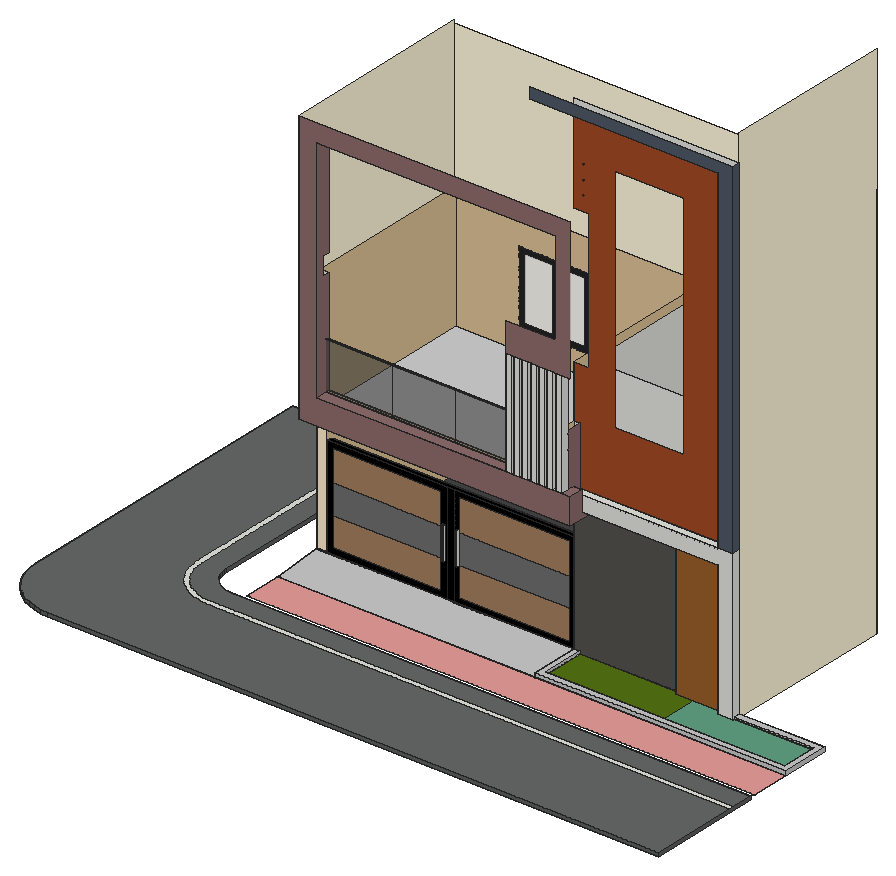
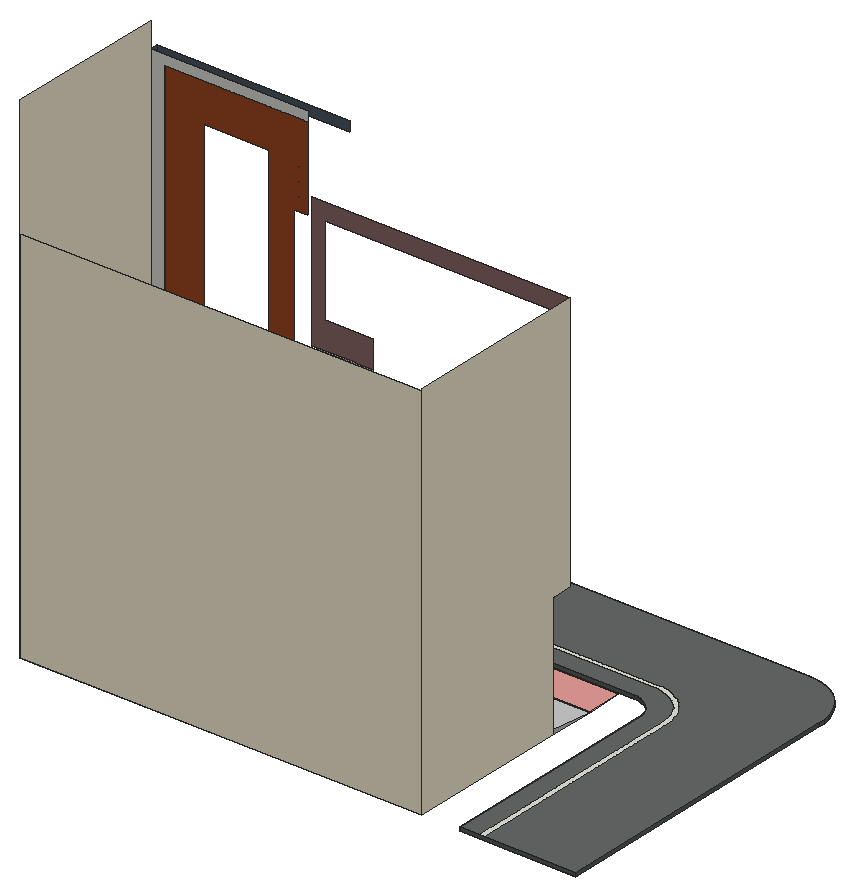
# SketchUp Ruby script. Lengths in inches.
U = 1.inch
M = Sketchup.active_model
def pt(a) = Geom::Point3d.new(a.map { |v| v * U })
def face(e, loops, mat)
  f = e.add_face(loops[0].map { |a| pt(a) })
  loops[1..].each { |l| e.add_face(l.map { |a| pt(a) }).erase! }
  f.material = f.back_material = mat if mat
  f
end
# faces: each face lists its corners as indices into pts; further lists are holes
def faces(e, pts, list, mat = nil) = list.each { |f| face(e, (f[0].is_a?(Array) ? f : [f]).map { |l| l.map { |i| pts[i] } }, mat) }
# xy, xz, yz: faces in a plane at the given z, y or x. An outline is a flat list of corners, or four numbers for a rectangle; further outlines are holes
def ring(l) = l.size == 4 ? [[l[0], l[1]], [l[2], l[1]], [l[2], l[3]], [l[0], l[3]]] : l.each_slice(2).to_a
def flat(e, list, mat, &to3) = list.each { |f| face(e, (f[0].is_a?(Array) ? f : [f]).map { |l| ring(l).map { |u, v| to3.(u, v) } }, mat) }
def xy(e, z, list, mat = nil) = flat(e, list, mat) { |x, y| [x, y, z] }
def xz(e, y, list, mat = nil) = flat(e, list, mat) { |x, z| [x, y, z] }
def yz(e, x, list, mat = nil) = flat(e, list, mat) { |y, z| [x, y, z] }
def lines(e, pts, list) = list.each { |a, b| e.add_line(pt(pts[a]), pt(pts[b])) }
# prism: a flat outline (further loops are holes) pulled along v
def prism(e, loops, v, mat = nil)
  f = face(e, loops, mat); d = Geom::Vector3d.new(v.map { |x| x * U })
  f.pushpull(f.normal.samedirection?(d) ? d.length : -d.length)
end
def box(e, o, s, mat = nil) = prism(e, [[o, [o[0] + s[0], o[1], o[2]], [o[0] + s[0], o[1] + s[1], o[2]], [o[0], o[1] + s[1], o[2]]]], [0, 0, s[2]], mat)
def at(x, y, z, deg = 0) = Geom::Transformation.translation(pt([x, y, z])) * Geom::Transformation.rotation(ORIGIN, Z_AXIS, deg.degrees)
def axes(o, x, y, z) = Geom::Transformation.new([*x, 0, *y, 0, *z, 0, *pt(o).to_a, 1])
def part(name) = M.definitions.add(name)
# library, detail: a bought-in or finely detailed component or shape, given as its bounding box
def library(name, o, s) = part(name).tap { |d| box(d.entities, o, s) }
def detail(e, o, s) = box(e.add_group.entities, o, s)
def put(e, d, t, mat = nil) = e.add_instance(d, t).tap { |i| i.material = mat if mat }
def group(e, t, mat = nil) = e.add_group.tap { |g| g.transformation = t; g.material = mat if mat }.entities
root = M.entities
M.materials.add("[0029_BlanchedAlmond]").color = [255, 235, 205]
M.materials.add("[0033_NavajoWhite]").color = [221, 193, 150]
M.materials.add("[0051_Cornsilk]").color = [255, 248, 220]
M.materials.add("[0111_SlateGray]").color = [79, 90, 102]
M.materials.add("[0119_RosyBrown]").color = [142, 108, 108]
M.materials.add("[0136_Charcoal]").color = [35, 35, 35]
M.materials.add("[0137_Black]").color = [0, 0, 0]
M.materials.add("[Blacktop Old 02]").color = [103, 104, 104]
M.materials.add("[Blacktop Old 02]1").color = [93, 94, 94]
M.materials.add("[Blacktop Old 02]2").color = [120, 122, 122]
M.materials.add("[Brick Basket]").color = [230, 156, 152]
M.materials.add("[Carrera Marble]").color = [207, 207, 207]
M.materials.add("[Cladding Siding Tan]").color = [162, 73, 37]
M.materials.add("[Cladding Siding Tan]1").color = [162, 126, 95]
M.materials.add("[Cladding Stucco White]").color = [198, 198, 198]
M.materials.add("[Granite Dark Gray]").color = [69, 68, 68]
M.materials.add("[Tile Travertine 2 inch]").color = [84, 82, 79]
M.materials.add("[Translucent Glass Gray]").color = [56, 56, 56]
M.materials["[Translucent Glass Gray]"].alpha = 0.5
M.materials.add("[Translucent Resin Crush Gray]").color = [249, 249, 249]
M.materials["[Translucent Resin Crush Gray]"].alpha = 0.8
M.materials.add("[Vegetation Blur 03]").color = [83, 114, 18]
M.materials.add("[Vegetation Ivy Hedera]").color = [97, 160, 130]
M.materials.add("[White Tile Black Accent]").color = [110, 110, 110]
M.materials.add("[Wood Cherry Original]").color = [152, 86, 42]
M.materials.add("[Wood Floor Dark]").color = [153, 94, 42]
box(root,[2453.375,1252.62,24],[816,852,720])
xy(root,-14,[[326.96,0,284.28,2.8,242.34,11.14,201.84,24.89,163.48,43.8,127.92,67.56,95.76,95.76,67.56,127.92,43.8,163.48,24.89,201.84,11.14,242.34,2.8,284.28,0,326.96,0,2165.125,700.8125,2165.125,700.8125,812.82,702.12,792.87,706.02,773.27,712.45,754.34,721.29,736.41,732.39,719.79,745.57,704.76,760.6,691.58,777.22,680.47,795.15,671.63,814.08,665.21,833.68,661.31,853.63,660,3833.375,660,3833.375,0]],"[Blacktop Old 02]2")
xy(root,0,[[917.375,690.18,3833.375,912.18],[917.375,912.18,2393.375,1192.62],[2393.375,912.18,2393.375,1192.62,2429.375,1192.62,2429.375,948.18,3797.375,948.18,3797.375,1156.62,3341.375,1156.62,3341.375,1192.62,3833.375,1192.62,3833.375,912.18],[2429.375,948.18,2429.375,1192.62,3341.375,1192.62,3341.375,1156.62,3797.375,1156.62,3797.375,948.18],[917.375,1192.62,3341.375,2176.62]])
xy(root,1,[[917.375,690.18,3833.375,912.18]],"[Brick Basket]")
xy(root,6,[[828.07,513.84,3833.375,513.84,3833.375,540,828.07,540,795.79,542.12,764.07,548.43,733.45,558.82,704.44,573.125,677.55,591.09,653.23,612.42,631.91,636.74,613.9375,663.63,599.63,692.63,589.24,723.26,582.93,754.98,580.8125,787.25,580.8125,2165.125,554.65,2165.125,554.65,787.25,556.99,751.57,563.97,716.49,575.46,682.625,591.28,650.55,611.15,620.81,634.73,593.92,661.62,570.34,691.36,550.47,723.4375,534.65,757.3,523.16,792.38,516.18]])
xy(root,6,[[326.96,0,3833.375,0,3833.375,513.84,828.07,513.84,792.38,516.18,757.3,523.16,723.4375,534.65,691.36,550.47,661.62,570.34,634.73,593.92,611.15,620.81,591.28,650.55,575.46,682.625,563.97,716.49,556.99,751.57,554.65,787.25,554.65,2165.125,0,2165.125,0,326.96,2.8,284.28,11.14,242.34,24.89,201.84,43.8,163.48,67.56,127.92,95.76,95.76,127.92,67.56,163.48,43.8,201.84,24.89,242.34,11.14,284.28,2.8],[828.07,540,3833.375,540,3833.375,660,853.63,660,833.68,661.31,814.08,665.21,795.15,671.63,777.22,680.47,760.6,691.58,745.57,704.76,732.39,719.79,721.29,736.41,712.45,754.34,706.02,773.27,702.12,792.87,700.8125,812.82,700.8125,2165.125,580.8125,2165.125,580.8125,787.25,582.93,754.98,589.24,723.26,599.63,692.63,613.9375,663.63,631.91,636.74,653.23,612.42,677.55,591.09,704.44,573.125,733.45,558.82,764.07,548.43,795.79,542.12]],"[Blacktop Old 02]")
xy(root,12,[[2429.375,948.18,3090.89,948.18,3090.89,1171.02,2993.375,1171.02,2993.375,1192.62,2429.375,1192.62]],"[Vegetation Blur 03]")
xy(root,12,[[3090.89,948.18,3797.375,948.18,3797.375,1156.62,3341.375,1156.62,3341.375,1144.62,3257.375,1144.62,3257.375,1171.02,3090.89,1171.02]],"[Vegetation Ivy Hedera]")
xy(root,12,[[2993.375,1171.02,3257.375,1192.62]],"[Wood Floor Dark]")
xy(root,24,[[1661.375,1188.18,1709.375,1192.62],[1709.375,1188.18,2393.375,1192.62],[977.375,1192.62,2393.375,1222.62]])
xy(root,24,[[917.375,1188.18,1661.375,1192.62]],"[Cladding Stucco White]")
xy(root,24,[[977.375,1222.62,2393.375,2104.62]],"[Granite Dark Gray]")
xy(root,25.2,[[2393.375,912.18,3833.375,912.18,3833.375,1192.62,3341.375,1192.62,3341.375,1156.62,3797.375,1156.62,3797.375,948.18,2429.375,948.18,2429.375,1192.62,2393.375,1192.62]],"[Cladding Stucco White]")
xy(root,216.33,[[1642.12,1181.62,1653.74,1192.62],[1718.31,1181.62,1729.93,1192.62]])
xy(root,400.83,[[1642.12,1181.62,1653.74,1192.62],[1718.31,1181.62,1729.93,1192.62]])
xy(root,600,[[977.375,1192.62,2393.375,1222.62]],"[0137_Black]")
xy(root,744,[[1171.92,1490.05,1169.42,1490.28,1166.95,1490.78,1164.56,1491.54,1162.25,1492.53,1160.0625,1493.77,1158.02,1495.23,1156.13,1496.89,1154.43,1498.74,1152.9375,1500.76,1151.66,1502.92,1150.62,1505.2,1149.82,1507.59,1149.27,1510.04,1148.98,1512.53,1148.96,1515.05,1149.2,1517.55,1149.69,1520.01,1150.45,1522.41,1151.45,1524.71,1152.68,1526.9,1154.14,1528.94,1155.8,1530.83,1157.65,1532.53,1159.67,1534.02,1161.83,1535.3,1164.12,1536.35,1166.5,1537.15,1168.95,1537.69,1171.44,1537.98,1173.96,1538,1176.46,1537.77,1178.92,1537.27,1181.32,1536.51,1183.62,1535.52,1185.81,1534.28,1187.86,1532.82,1189.74,1531.16,1191.4375,1529.3125,1192.93,1527.29,1194.21,1525.13,1195.26,1522.85,1196.06,1520.46,1196.6,1518.01,1196.89,1515.52,1196.91,1513.01,1196.68,1510.5,1196.18,1508.04,1195.43,1505.65,1194.43,1503.34,1193.19,1501.15,1191.74,1499.11,1190.07,1497.22,1188.22,1495.52,1186.21,1494.03,1184.04,1492.75,1181.76,1491.71,1179.375,1490.91,1176.92,1490.36,1174.43,1490.07],[1615.92,1490.05,1613.42,1490.28,1610.95,1490.78,1608.56,1491.54,1606.25,1492.53,1604.0625,1493.77,1602.02,1495.23,1600.13,1496.89,1598.43,1498.74,1596.9375,1500.76,1595.66,1502.92,1594.62,1505.2,1593.82,1507.59,1593.27,1510.04,1592.98,1512.53,1592.96,1515.05,1593.2,1517.55,1593.69,1520.01,1594.45,1522.41,1595.45,1524.71,1596.68,1526.9,1598.14,1528.94,1599.8,1530.83,1601.65,1532.53,1603.67,1534.02,1605.83,1535.3,1608.12,1536.35,1610.5,1537.15,1612.95,1537.69,1615.44,1537.98,1617.96,1538,1620.46,1537.77,1622.92,1537.27,1625.32,1536.51,1627.62,1535.52,1629.81,1534.28,1631.86,1532.82,1633.74,1531.16,1635.4375,1529.3125,1636.93,1527.29,1638.21,1525.13,1639.26,1522.85,1640.06,1520.46,1640.6,1518.01,1640.89,1515.52,1640.91,1513.01,1640.68,1510.5,1640.18,1508.04,1639.43,1505.65,1638.43,1503.34,1637.19,1501.15,1635.74,1499.11,1634.07,1497.22,1632.22,1495.52,1630.21,1494.03,1628.04,1492.75,1625.76,1491.71,1623.375,1490.91,1620.92,1490.36,1618.43,1490.07],[2059.92,1490.05,2057.42,1490.28,2054.95,1490.78,2052.56,1491.54,2050.25,1492.53,2048.0625,1493.77,2046.02,1495.23,2044.13,1496.89,2042.43,1498.74,2040.9375,1500.76,2039.66,1502.92,2038.62,1505.2,2037.82,1507.59,2037.27,1510.04,2036.98,1512.53,2036.96,1515.05,2037.2,1517.55,2037.69,1520.01,2038.45,1522.41,2039.45,1524.71,2040.68,1526.9,2042.14,1528.94,2043.8,1530.83,2045.65,1532.53,2047.67,1534.02,2049.83,1535.3,2052.12,1536.35,2054.5,1537.15,2056.95,1537.69,2059.44,1537.98,2061.96,1538,2064.46,1537.77,2066.92,1537.27,2069.32,1536.51,2071.62,1535.52,2073.81,1534.28,2075.86,1532.82,2077.74,1531.16,2079.4375,1529.3125,2080.93,1527.29,2082.21,1525.13,2083.26,1522.85,2084.06,1520.46,2084.6,1518.01,2084.89,1515.52,2084.91,1513.01,2084.68,1510.5,2084.18,1508.04,2083.43,1505.65,2082.43,1503.34,2081.19,1501.15,2079.74,1499.11,2078.07,1497.22,2076.22,1495.52,2074.21,1494.03,2072.04,1492.75,2069.76,1491.71,2067.375,1490.91,2064.92,1490.36,2062.43,1490.07]])
xy(root,744,[[[977.375,1060.62,977.375,2104.62,2393.375,2104.62,2393.375,1192.62,2477.375,1192.62,2477.375,1060.62],[1615.92,1490.05,1618.43,1490.07,1620.92,1490.36,1623.375,1490.91,1625.76,1491.71,1628.04,1492.75,1630.21,1494.03,1632.22,1495.52,1634.07,1497.22,1635.74,1499.11,1637.19,1501.15,1638.43,1503.34,1639.43,1505.65,1640.18,1508.04,1640.68,1510.5,1640.91,1513.01,1640.89,1515.52,1640.6,1518.01,1640.06,1520.46,1639.26,1522.85,1638.21,1525.13,1636.93,1527.29,1635.4375,1529.3125,1633.74,1531.16,1631.86,1532.82,1629.81,1534.28,1627.62,1535.52,1625.32,1536.51,1622.92,1537.27,1620.46,1537.77,1617.96,1538,1615.44,1537.98,1612.95,1537.69,1610.5,1537.15,1608.12,1536.35,1605.83,1535.3,1603.67,1534.02,1601.65,1532.53,1599.8,1530.83,1598.14,1528.94,1596.68,1526.9,1595.45,1524.71,1594.45,1522.41,1593.69,1520.01,1593.2,1517.55,1592.96,1515.05,1592.98,1512.53,1593.27,1510.04,1593.82,1507.59,1594.62,1505.2,1595.66,1502.92,1596.9375,1500.76,1598.43,1498.74,1600.13,1496.89,1602.02,1495.23,1604.0625,1493.77,1606.25,1492.53,1608.56,1491.54,1610.95,1490.78,1613.42,1490.28],[2059.92,1490.05,2062.43,1490.07,2064.92,1490.36,2067.375,1490.91,2069.76,1491.71,2072.04,1492.75,2074.21,1494.03,2076.22,1495.52,2078.07,1497.22,2079.74,1499.11,2081.19,1501.15,2082.43,1503.34,2083.43,1505.65,2084.18,1508.04,2084.68,1510.5,2084.91,1513.01,2084.89,1515.52,2084.6,1518.01,2084.06,1520.46,2083.26,1522.85,2082.21,1525.13,2080.93,1527.29,2079.4375,1529.3125,2077.74,1531.16,2075.86,1532.82,2073.81,1534.28,2071.62,1535.52,2069.32,1536.51,2066.92,1537.27,2064.46,1537.77,2061.96,1538,2059.44,1537.98,2056.95,1537.69,2054.5,1537.15,2052.12,1536.35,2049.83,1535.3,2047.67,1534.02,2045.65,1532.53,2043.8,1530.83,2042.14,1528.94,2040.68,1526.9,2039.45,1524.71,2038.45,1522.41,2037.69,1520.01,2037.2,1517.55,2036.96,1515.05,2036.98,1512.53,2037.27,1510.04,2037.82,1507.59,2038.62,1505.2,2039.66,1502.92,2040.9375,1500.76,2042.43,1498.74,2044.13,1496.89,2046.02,1495.23,2048.0625,1493.77,2050.25,1492.53,2052.56,1491.54,2054.95,1490.78,2057.42,1490.28],[1171.92,1490.05,1174.43,1490.07,1176.92,1490.36,1179.375,1490.91,1181.76,1491.71,1184.04,1492.75,1186.21,1494.03,1188.22,1495.52,1190.07,1497.22,1191.74,1499.11,1193.19,1501.15,1194.43,1503.34,1195.43,1505.65,1196.18,1508.04,1196.68,1510.5,1196.91,1513.01,1196.89,1515.52,1196.6,1518.01,1196.06,1520.46,1195.26,1522.85,1194.21,1525.13,1192.93,1527.29,1191.4375,1529.3125,1189.74,1531.16,1187.86,1532.82,1185.81,1534.28,1183.62,1535.52,1181.32,1536.51,1178.92,1537.27,1176.46,1537.77,1173.96,1538,1171.44,1537.98,1168.95,1537.69,1166.5,1537.15,1164.12,1536.35,1161.83,1535.3,1159.67,1534.02,1157.65,1532.53,1155.8,1530.83,1154.14,1528.94,1152.68,1526.9,1151.45,1524.71,1150.45,1522.41,1149.69,1520.01,1149.2,1517.55,1148.96,1515.05,1148.98,1512.53,1149.27,1510.04,1149.82,1507.59,1150.62,1505.2,1151.66,1502.92,1152.9375,1500.76,1154.43,1498.74,1156.13,1496.89,1158.02,1495.23,1160.0625,1493.77,1162.25,1492.53,1164.56,1491.54,1166.95,1490.78,1169.42,1490.28]]],"[0033_NavajoWhite]")
xy(root,744,[[917.375,1060.62,977.375,1192.62]],"[0119_RosyBrown]")
xy(root,780,[[2393.375,1144.62,2477.375,1192.62],[2477.375,1144.62,2477.375,1192.62,2993.375,1192.62,2993.375,1171.02,3257.375,1171.02,3257.375,1144.62],[2453.375,1252.62,3281.375,2116.62]])
xy(root,780,[[977.375,1144.62,2393.375,2116.62]],"[Carrera Marble]")
xy(root,780,[[2993.375,1171.02,3257.375,1192.62]],"[Wood Floor Dark]")
xy(root,864,[[2427.51,1144.62,3257.375,1192.62],[3257.375,1144.62,3341.375,1192.62]])
xy(root,894,[[2105.375,1060.62,2139.51,1102.62],[2139.51,1060.62,2153.375,1102.62],[2153.375,1060.62,2187.51,1102.62],[2187.51,1060.62,2201.375,1102.62],[2201.375,1060.62,2235.51,1102.62],
  [2235.51,1060.62,2249.375,1102.62],[2249.375,1060.62,2283.51,1102.62],[2283.51,1060.62,2297.375,1102.62],[2297.375,1060.62,2331.51,1102.62],[2331.51,1060.62,2345.375,1102.62],
  [2345.375,1060.62,2379.51,1102.62],[2379.51,1060.62,2393.375,1102.62],[2393.375,1060.62,2427.51,1102.62],[2393.375,1102.62,2427.51,1144.62]])
xy(root,894,[[1025.375,1123.62,2393.375,1144.62]],"[0033_NavajoWhite]")
xy(root,894,[[1025.375,1060.62,2105.375,1060.62,2105.375,1102.62,2393.375,1102.62,2393.375,1123.62,1025.375,1123.62],[2427.51,1060.62,2477.375,1144.62]],"[0119_RosyBrown]")
xz(root,0,[[326.96,-14,3833.375,6]],"[Blacktop Old 02]1")
xz(root,660,[[853.63,-14,3833.375,6]],"[Blacktop Old 02]1")
xz(root,690.18,[[917.375,0,3833.375,1]])
xz(root,912.18,[[917.375,0,2393.375,1],[2393.375,0,3833.375,1]])
xz(root,912.18,[[2393.375,1,3833.375,25.2]],"[Cladding Stucco White]")
xz(root,948.18,[[2429.375,0,3797.375,12]])
xz(root,948.18,[[2429.375,12,3797.375,25.2]],"[Cladding Stucco White]")
xz(root,1060.62,[[2105.375,894,2139.51,1500],[2153.375,894,2187.51,1500],[2201.375,894,2235.51,1500],[2249.375,894,2283.51,1500],[2297.375,894,2331.51,1500],
  [2345.375,894,2379.51,1500],[2393.375,894,2427.51,1500]])
xz(root,1060.62,[[917.375,744,2477.375,744,2477.375,894,1025.375,894,1025.375,2203,2393.375,2203,2393.375,1668,2105.375,1668,2105.375,1500,2477.375,1500,2477.375,2305.2,917.375,2305.2]],"[0119_RosyBrown]")
xz(root,1102.62,[[2105.375,894,2139.51,1500],[2153.375,894,2187.51,1500],[2201.375,894,2235.51,1500],[2249.375,894,2283.51,1500],[2297.375,894,2331.51,1500],
  [2345.375,894,2379.51,1500],[2393.375,894,2427.51,1197]])
xz(root,1123.62,[[1025.375,1166,2393.375,1170]])
xz(root,1123.62,[[1025.375,894,1409.375,1166],[1409.375,894,1769.375,1166],[1769.375,894,2393.375,1166]],"[Translucent Glass Gray]")
xz(root,1144.62,[[3257.375,12,3341.375,12,3341.375,864,2477.375,864,2477.375,780,3257.375,780],[977.375,780,1025.375,1500],[2393.375,780,2477.375,864],[2393.375,864,2427.51,894],[2427.51,864,2477.375,894]])
xz(root,1144.62,[[1025.375,780,2393.375,894]],"[0033_NavajoWhite]")
xz(root,1144.62,[[3257.375,864,3341.375,864,3341.375,2856,2177.375,2856,2177.375,2796,3257.375,2796]],"[0111_SlateGray]")
xz(root,1156.62,[[3341.375,0,3797.375,12]])
xz(root,1156.62,[[3341.375,12,3797.375,25.2]],"[Cladding Stucco White]")
xz(root,1171.02,[[2993.375,12,3257.375,780]],"[Wood Floor Dark]")
xz(root,1181.62,[[1642.12,216.33,1653.74,400.83],[1718.31,216.33,1729.93,400.83]])
xz(root,1192.62,[[917.375,0,2393.375,24],[2393.375,0,2429.375,25.2],[3257.375,0,3257.375,780,2393.375,780,2393.375,864,3341.375,864,3341.375,0],[2429.375,0,2993.375,12],[2993.375,0,3257.375,12],
  [3341.375,0,3833.375,25.2],[2393.375,864,2427.51,1197],[3257.375,864,3257.375,2796,2393.375,2796,2393.375,2856,3341.375,2856,3341.375,864]])
xz(root,1192.62,[[917.375,24,977.375,744]],"[0029_BlanchedAlmond]")
xz(root,1192.62,[[[977.375,24,1661.375,600],[1007.375,54,1631.375,570],[1642.12,216.33,1653.74,400.83]],[1661.375,24,1709.375,600],[[1709.375,24,2393.375,600],[1739.375,54,2363.375,570],[1718.31,216.33,1729.93,400.83]]],"[0137_Black]")
xz(root,1192.62,[[[2427.51,864,3257.375,864,3257.375,2796,2393.375,2796,2393.375,2292,2477.375,2292,2477.375,1500,2393.375,1500,2393.375,1197,2427.51,1197],[2627.375,1242,3023.375,2562],[2448.125,2446,2447.29,2446.04,2446.46,2446.17,2445.65,2446.39,2444.87,2446.69,2444.125,2447.07,2443.42,2447.53,2442.77,2448.05,2442.18,2448.65,2441.65,2449.3,2441.19,2450,2440.81,2450.75,2440.51,2451.53,2440.3,2452.34,2440.17,2453.16,2440.125,2454,2440.17,2454.84,2440.3,2455.66,2440.51,2456.47,2440.81,2457.25,2441.19,2458,2441.65,2458.7,2442.18,2459.35,2442.77,2459.95,2443.42,2460.47,2444.125,2460.93,2444.87,2461.31,2445.65,2461.61,2446.46,2461.83,2447.29,2461.96,2448.125,2462,2448.96,2461.96,2449.79,2461.83,2450.6,2461.61,2451.38,2461.31,2452.125,2460.93,2452.83,2460.47,2453.48,2459.95,2454.07,2459.35,2454.6,2458.7,2455.05,2458,2455.43,2457.25,2455.73,2456.47,2455.95,2455.66,2456.08,2454.84,2456.125,2454,2456.08,2453.16,2455.95,2452.34,2455.73,2451.53,2455.43,2450.75,2455.05,2450,2454.6,2449.3,2454.07,2448.65,2453.48,2448.05,2452.83,2447.53,2452.125,2447.07,2451.38,2446.69,2450.6,2446.39,2449.79,2446.17,2448.96,2446.04],[2448.125,2365,2447.29,2365.04,2446.46,2365.17,2445.65,2365.39,2444.87,2365.69,2444.125,2366.07,2443.42,2366.53,2442.77,2367.05,2442.18,2367.65,2441.65,2368.3,2441.19,2369,2440.81,2369.75,2440.51,2370.53,2440.3,2371.34,2440.17,2372.16,2440.125,2373,2440.17,2373.84,2440.3,2374.66,2440.51,2375.47,2440.81,2376.25,2441.19,2377,2441.65,2377.7,2442.18,2378.35,2442.77,2378.95,2443.42,2379.47,2444.125,2379.93,2444.87,2380.31,2445.65,2380.61,2446.46,2380.83,2447.29,2380.96,2448.125,2381,2448.96,2380.96,2449.79,2380.83,2450.6,2380.61,2451.38,2380.31,2452.125,2379.93,2452.83,2379.47,2453.48,2378.95,2454.07,2378.35,2454.6,2377.7,2455.05,2377,2455.43,2376.25,2455.73,2375.47,2455.95,2374.66,2456.08,2373.84,2456.125,2373,2456.08,2372.16,2455.95,2371.34,2455.73,2370.53,2455.43,2369.75,2455.05,2369,2454.6,2368.3,2454.07,2367.65,2453.48,2367.05,2452.83,2366.53,2452.125,2366.07,2451.38,2365.69,2450.6,2365.39,2449.79,2365.17,2448.96,2365.04],[2448.125,2527,2447.29,2527.04,2446.46,2527.17,2445.65,2527.39,2444.87,2527.69,2444.125,2528.07,2443.42,2528.53,2442.77,2529.05,2442.18,2529.65,2441.65,2530.3,2441.19,2531,2440.81,2531.75,2440.51,2532.53,2440.3,2533.34,2440.17,2534.16,2440.125,2535,2440.17,2535.84,2440.3,2536.66,2440.51,2537.47,2440.81,2538.25,2441.19,2539,2441.65,2539.7,2442.18,2540.35,2442.77,2540.95,2443.42,2541.47,2444.125,2541.93,2444.87,2542.31,2445.65,2542.61,2446.46,2542.83,2447.29,2542.96,2448.125,2543,2448.96,2542.96,2449.79,2542.83,2450.6,2542.61,2451.38,2542.31,2452.125,2541.93,2452.83,2541.47,2453.48,2540.95,2454.07,2540.35,2454.6,2539.7,2455.05,2539,2455.43,2538.25,2455.73,2537.47,2455.95,2536.66,2456.08,2535.84,2456.125,2535,2456.08,2534.16,2455.95,2533.34,2455.73,2532.53,2455.43,2531.75,2455.05,2531,2454.6,2530.3,2454.07,2529.65,2453.48,2529.05,2452.83,2528.53,2452.125,2528.07,2451.38,2527.69,2450.6,2527.39,2449.79,2527.17,2448.96,2527.04]]],"[Cladding Siding Tan]")
xz(root,1192.62,[[1007.375,54,1631.375,222],[1739.375,54,2363.375,222],[1007.375,390,1631.375,570],[1739.375,390,2363.375,570]],"[Cladding Siding Tan]1")
xz(root,1192.62,[[2429.375,12,2993.375,12,2993.375,780,2477.375,780,2477.375,744,2393.375,744,2393.375,25.2,2429.375,25.2]],"[Tile Travertine 2 inch]")
xz(root,1192.62,[[1007.375,222,1631.375,390],[1739.375,222,2363.375,390]],"[White Tile Black Accent]")
xz(root,1222.62,[[977.375,24,2393.375,600]],"[Cladding Siding Tan]1")
xz(root,1252.62,[[2453.375,780,3281.375,1500]])
xz(root,2104.62,[[977.375,24,2393.375,744]],"[0033_NavajoWhite]")
xz(root,2116.62,[[2453.375,780,3281.375,1500]])
xz(root,2116.62,[[[977.375,780,2393.375,1500],[1339.41,901.56,1744.91,1319.81]]],"[0033_NavajoWhite]")
xz(root,2116.62,[[[1339.41,901.56,1744.91,1319.81],[1369.41,931.56,1530.16,1289.81],[1554.16,931.56,1714.91,1289.81]]],"[0136_Charcoal]")
xz(root,2116.62,[[1369.41,931.56,1530.16,1289.81],[1554.16,931.56,1714.91,1289.81]],"[Translucent Resin Crush Gray]")
xz(root,2165.125,[[0,-14,700.8125,6]],"[Blacktop Old 02]1")
xz(root,2176.62,[[917.375,0,3341.375,2292]],"[0051_Cornsilk]")
yz(root,0,[[326.96,-14,2165.125,6]],"[Blacktop Old 02]1")
yz(root,700.8125,[[812.82,-14,2165.125,6]],"[Blacktop Old 02]1")
yz(root,917.375,[[690.18,0,912.18,1]])
yz(root,917.375,[[1192.62,0,1192.62,744,1060.62,744,1060.62,2305.2,2176.62,2305.2,2176.62,0]],"[0051_Cornsilk]")
yz(root,917.375,[[912.18,0,1188.18,24,1192.62,24,1192.62,0]],"[Cladding Stucco White]")
yz(root,977.375,[[1192.62,24,1222.62,600]])
yz(root,977.375,[[1222.62,24,2104.62,24,2104.62,744,1192.62,744,1192.62,600,1222.62,600],[1144.62,780,2116.62,1500]],"[0033_NavajoWhite]")
yz(root,1025.375,[[1123.62,1166,1122.58,1166.14,1121.62,1166.54,1120.79,1167.17,1120.15,1168,1119.75,1168.96,1119.62,1170,1119.75,1171.04,1120.15,1172,1120.79,1172.83,1121.62,1173.46,1122.58,1173.86,1123.62,1174,1124.65,1173.86,1125.62,1173.46,1126.45,1172.83,1127.08,1172,1127.48,1171.04,1127.62,1170,1127.48,1168.96,1127.08,1168,1126.45,1167.17,1125.62,1166.54,1124.65,1166.14]])
yz(root,1025.375,[[[1060.62,894,1144.62,894,1144.62,1500,1102.62,1500,1102.62,1602,1144.62,1602,1144.62,2203,1060.62,2203],[1123.62,1166,1122.58,1166.14,1121.62,1166.54,1120.79,1167.17,1120.15,1168,1119.75,1168.96,1119.62,1170,1119.75,1171.04,1120.15,1172,1120.79,1172.83,1121.62,1173.46,1122.58,1173.86,1123.62,1174,1124.65,1173.86,1125.62,1173.46,1126.45,1172.83,1127.08,1172,1127.48,1171.04,1127.62,1170,1127.48,1168.96,1127.08,1168,1126.45,1167.17,1125.62,1166.54,1124.65,1166.14],[1123.62,1826,1122.58,1826.14,1121.62,1826.54,1120.79,1827.17,1120.15,1828,1119.75,1828.96,1119.62,1830,1119.75,1831.04,1120.15,1832,1120.79,1832.83,1121.62,1833.46,1122.58,1833.86,1123.62,1834,1124.65,1833.86,1125.62,1833.46,1126.45,1832.83,1127.08,1832,1127.48,1831.04,1127.62,1830,1127.48,1828.96,1127.08,1828,1126.45,1827.17,1125.62,1826.54,1124.65,1826.14]]],"[0119_RosyBrown]")
yz(root,1642.12,[[1181.62,216.33,1192.62,400.83]])
yz(root,1653.74,[[1181.62,216.33,1192.62,400.83]])
yz(root,1718.31,[[1181.62,216.33,1192.62,400.83]])
yz(root,1729.93,[[1181.62,216.33,1192.62,400.83]])
yz(root,2105.375,[[1060.62,894,1102.62,1500]])
yz(root,2139.51,[[1060.62,894,1102.62,1500]])
yz(root,2153.375,[[1060.62,894,1102.62,1500]])
yz(root,2187.51,[[1060.62,894,1102.62,1500]])
yz(root,2201.375,[[1060.62,894,1102.62,1500]])
yz(root,2235.51,[[1060.62,894,1102.62,1500]])
yz(root,2249.375,[[1060.62,894,1102.62,1500]])
yz(root,2283.51,[[1060.62,894,1102.62,1500]])
yz(root,2297.375,[[1060.62,894,1102.62,1500]])
yz(root,2331.51,[[1060.62,894,1102.62,1500]])
yz(root,2345.375,[[1060.62,894,1102.62,1500]])
yz(root,2379.51,[[1060.62,894,1102.62,1500]])
yz(root,2393.375,[[912.18,0,1188.18,24,1192.62,24,1192.62,0],[1192.62,24,1222.62,600],[1060.62,894,1102.62,1500]])
yz(root,2393.375,[[[1144.62,780,1144.62,894,1102.62,894,1102.62,1197,1192.62,1197,1192.62,780],[1123.62,1166,1124.65,1166.14,1125.62,1166.54,1126.45,1167.17,1127.08,1168,1127.48,1168.96,1127.62,1170,1127.48,1171.04,1127.08,1172,1126.45,1172.83,1125.62,1173.46,1124.65,1173.86,1123.62,1174,1122.58,1173.86,1121.62,1173.46,1120.79,1172.83,1120.15,1172,1119.75,1171.04,1119.62,1170,1119.75,1168.96,1120.15,1168,1120.79,1167.17,1121.62,1166.54,1122.58,1166.14]],[1192.62,780,2116.62,1500]],"[0033_NavajoWhite]")
yz(root,2393.375,[[912.18,0,912.18,25.2,1192.62,25.2,1192.62,24,1188.18,24]],"[Cladding Stucco White]")
yz(root,2393.375,[[1222.62,24,1222.62,600,1192.62,600,1192.62,744,2104.62,744,2104.62,24]],"[Wood Cherry Original]")
yz(root,2427.51,[[1060.62,894,1102.62,1500]])
yz(root,2427.51,[[1144.62,864,1192.62,864,1192.62,1197,1102.62,1197,1102.62,894,1144.62,894]],"[0119_RosyBrown]")
yz(root,2429.375,[[948.18,0,1192.62,12]])
yz(root,2429.375,[[948.18,12,1192.62,25.2]],"[Cladding Stucco White]")
yz(root,2453.375,[[1252.62,780,2116.62,1500]])
yz(root,2477.375,[[1060.62,744,1192.62,744,1192.62,780,1144.62,780,1144.62,894,1060.62,894]],"[0119_RosyBrown]")
yz(root,2993.375,[[1171.02,12,1192.62,780]],"[Wood Floor Dark]")
yz(root,3257.375,[[1144.62,12,1171.02,780]])
yz(root,3257.375,[[1144.62,864,1192.62,2796]],"[0111_SlateGray]")
yz(root,3257.375,[[1171.02,12,1192.62,780]],"[Wood Floor Dark]")
yz(root,3281.375,[[1252.62,780,2116.62,1500]])
yz(root,3341.375,[[1156.62,0,1192.62,25.2],[1144.62,12,1156.62,12,1156.62,25.2,1192.62,25.2,1192.62,864,1144.62,864]])
yz(root,3341.375,[[1192.62,0,2176.62,3012]],"[0051_Cornsilk]")
yz(root,3341.375,[[1144.62,864,1192.62,2856]],"[0111_SlateGray]")
yz(root,3797.375,[[948.18,0,1156.62,12]])
yz(root,3797.375,[[948.18,12,1156.62,25.2]],"[Cladding Stucco White]")
yz(root,3833.375,[[690.18,0,912.18,1]])
yz(root,3833.375,[[0,-14,660,6]],"[Blacktop Old 02]1")
yz(root,3833.375,[[912.18,0,1192.62,25.2]],"[Cladding Stucco White]")
p = [[284.28,2.8,6],[284.28,2.8,-14],[326.96,0,-14],[326.96,0,6],[242.34,11.14,6],[242.34,11.14,-14],
  [201.84,24.89,6],[201.84,24.89,-14],[163.48,43.8,6],[163.48,43.8,-14],[127.92,67.56,6],[127.92,67.56,-14],
  [95.76,95.76,6],[95.76,95.76,-14],[67.56,127.92,6],[67.56,127.92,-14],[43.8,163.48,6],[43.8,163.48,-14],
  [24.89,201.84,6],[24.89,201.84,-14],[11.14,242.34,6],[11.14,242.34,-14],[2.8,284.28,6],[2.8,284.28,-14],
  [0,326.96,6],[0,326.96,-14],[853.63,660,6],[853.63,660,-14],[833.68,661.31,-14],[833.68,661.31,6],
  [814.08,665.21,-14],[814.08,665.21,6],[795.15,671.63,-14],[795.15,671.63,6],[777.22,680.47,-14],[777.22,680.47,6],
  [760.6,691.58,-14],[760.6,691.58,6],[745.57,704.76,-14],[745.57,704.76,6],[732.39,719.79,-14],[732.39,719.79,6],
  [721.29,736.41,-14],[721.29,736.41,6],[712.45,754.34,-14],[712.45,754.34,6],[706.02,773.27,-14],[706.02,773.27,6],
  [702.12,792.87,-14],[702.12,792.87,6],[700.8125,812.82,-14],[700.8125,812.82,6],[2393.375,912.18,0],[2393.375,1188.18,24],
  [1709.375,1188.18,24],[1661.375,1188.18,24],[917.375,1188.18,24],[917.375,912.18,0],[1025.375,1122.58,1166.14],[1025.375,1123.62,1166],
  [1409.375,1123.62,1166],[1769.375,1123.62,1166],[2393.375,1123.62,1166],[2393.375,1122.58,1166.14],[1025.375,1124.65,1166.14],[2393.375,1124.65,1166.14],
  [1025.375,1121.62,1166.54],[2393.375,1121.62,1166.54],[1025.375,1125.62,1166.54],[2393.375,1125.62,1166.54],[1025.375,1120.79,1167.17],[2393.375,1120.79,1167.17],
  [1025.375,1126.45,1167.17],[2393.375,1126.45,1167.17],[1025.375,1120.15,1168],[2393.375,1120.15,1168],[1025.375,1127.08,1168],[2393.375,1127.08,1168],
  [1025.375,1119.75,1168.96],[2393.375,1119.75,1168.96],[1025.375,1127.48,1168.96],[2393.375,1127.48,1168.96],[2393.375,2104.62,24],[2453.375,2104.62,24],
  [2393.375,2104.62,744],[2453.375,2104.62,744]]
faces(root,p,[[0,1,2,3],[4,5,1,0],[6,7,5,4],[8,9,7,6],[10,11,9,8],[12,13,11,10],[14,15,13,12],[16,17,15,14],
  [18,19,17,16],[20,21,19,18],[22,23,21,20],[24,25,23,22],[26,27,28,29],[29,28,30,31],[31,30,32,33],[33,32,34,35],
  [35,34,36,37],[37,36,38,39],[39,38,40,41],[41,40,42,43],[43,42,44,45],[45,44,46,47],[47,46,48,49],[49,48,50,51]],"[Blacktop Old 02]1")
faces(root,p,[[52,53,54,55,56,57]],"[Cladding Stucco White]")
faces(root,p,[[58,59,60,61,62,63],[59,64,65,62,61,60],[66,58,63,67],[64,68,69,65],[70,66,67,71],[68,72,73,69],[74,70,71,75],[72,76,77,73],
  [78,74,75,79],[76,80,81,77]],"[0136_Charcoal]")
lines(root,p,[[82,83],[84,85]])
